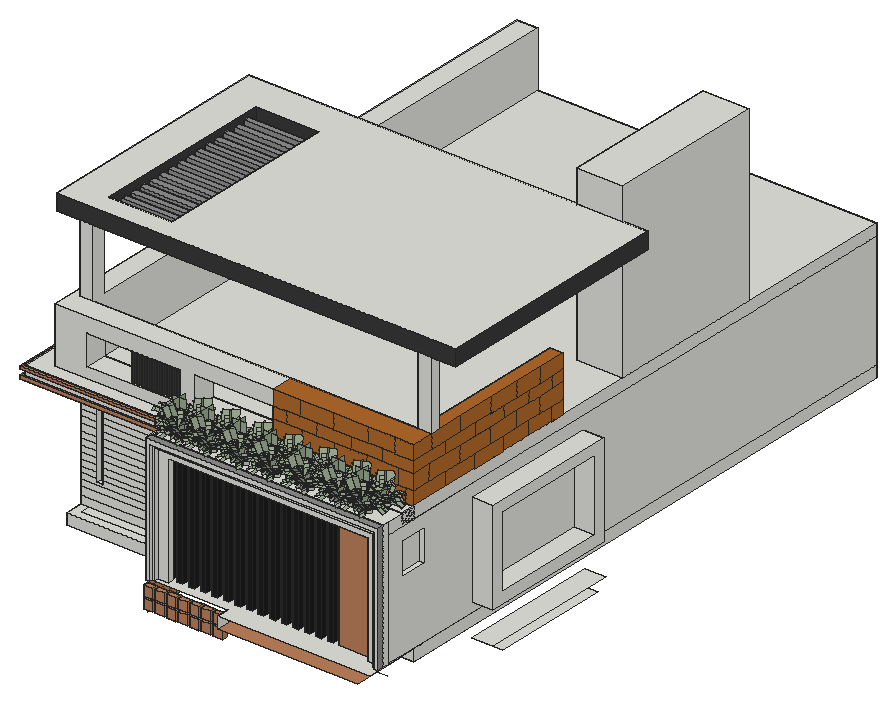
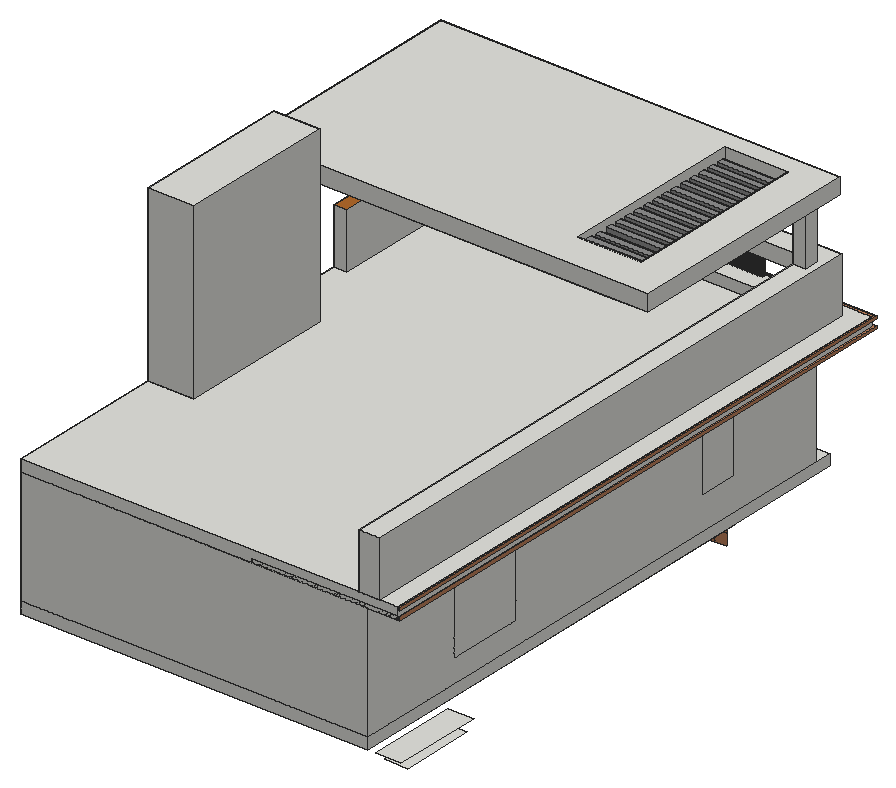
# SketchUp Ruby script. Lengths in inches.
U = 1.inch
M = Sketchup.active_model
def pt(a) = Geom::Point3d.new(a.map { |v| v * U })
def face(e, loops, mat)
  f = e.add_face(loops[0].map { |a| pt(a) })
  loops[1..].each { |l| e.add_face(l.map { |a| pt(a) }).erase! }
  f.material = f.back_material = mat if mat
  f
end
# faces: each face lists its corners as indices into pts; further lists are holes
def faces(e, pts, list, mat = nil) = list.each { |f| face(e, (f[0].is_a?(Array) ? f : [f]).map { |l| l.map { |i| pts[i] } }, mat) }
# xy, xz, yz: faces in a plane at the given z, y or x. An outline is a flat list of corners, or four numbers for a rectangle; further outlines are holes
def ring(l) = l.size == 4 ? [[l[0], l[1]], [l[2], l[1]], [l[2], l[3]], [l[0], l[3]]] : l.each_slice(2).to_a
def flat(e, list, mat, &to3) = list.each { |f| face(e, (f[0].is_a?(Array) ? f : [f]).map { |l| ring(l).map { |u, v| to3.(u, v) } }, mat) }
def xy(e, z, list, mat = nil) = flat(e, list, mat) { |x, y| [x, y, z] }
def xz(e, y, list, mat = nil) = flat(e, list, mat) { |x, z| [x, y, z] }
def yz(e, x, list, mat = nil) = flat(e, list, mat) { |y, z| [x, y, z] }
def lines(e, pts, list) = list.each { |a, b| e.add_line(pt(pts[a]), pt(pts[b])) }
# prism: a flat outline (further loops are holes) pulled along v
def prism(e, loops, v, mat = nil)
  f = face(e, loops, mat); d = Geom::Vector3d.new(v.map { |x| x * U })
  f.pushpull(f.normal.samedirection?(d) ? d.length : -d.length)
end
def box(e, o, s, mat = nil) = prism(e, [[o, [o[0] + s[0], o[1], o[2]], [o[0] + s[0], o[1] + s[1], o[2]], [o[0], o[1] + s[1], o[2]]]], [0, 0, s[2]], mat)
def at(x, y, z, deg = 0) = Geom::Transformation.translation(pt([x, y, z])) * Geom::Transformation.rotation(ORIGIN, Z_AXIS, deg.degrees)
def axes(o, x, y, z) = Geom::Transformation.new([*x, 0, *y, 0, *z, 0, *pt(o).to_a, 1])
def part(name) = M.definitions.add(name)
# library, detail: a bought-in or finely detailed component or shape, given as its bounding box
def library(name, o, s) = part(name).tap { |d| box(d.entities, o, s) }
def detail(e, o, s) = box(e.add_group.entities, o, s)
def put(e, d, t, mat = nil) = e.add_instance(d, t).tap { |i| i.material = mat if mat }
def group(e, t, mat = nil) = e.add_group.tap { |g| g.transformation = t; g.material = mat if mat }.entities
root = M.entities
M.materials.add("[Color M04]").color = [142, 142, 142]
M.materials.add("[Color M07]").color = [58, 58, 58]
M.materials.add("[Color M08]").color = [30, 30, 30]
M.materials.add("[Wood Bamboo]").color = [177, 105, 43]
M.materials.add("[Wood Veneer 02]").color = [190, 128, 91]
M.materials.add("hymenocallis littoralis").color = [156, 172, 146]
c1 = part("グループ\#88")
detail(c1.entities,[0,0,0],[11.8125,11.8125,1.69])
c2 = part("CL OL251733")
put(c2.entities,c1,axes([4.91,11.8125,72.56],[1,0,0],[0,-1,0],[0,0,-1]))
c3 = part("Group\#48")
box(c3.entities,[0,0,0],[5.9375,5.0625,120])
c4 = part("Group\#856")
xy(c4.entities,7.38,[[0,0,5.5,15.91]],"hymenocallis littoralis")
p = [[5.5,28.78,0],[5.5,26.79,3.44],[0,26.79,3.44],[0,28.78,0],[0,23.75,6],[5.5,23.75,6],
  [0,15.91,7.38],[5.5,15.91,7.38]]
faces(c4.entities,p,[[0,1,2,3],[4,2,1,5],[6,4,5,7]],"hymenocallis littoralis")
c5 = part("Group\#854")
xy(c5.entities,7.38,[[0,0,5.5,15.91],[0,15.91,5.5,23.87]],"hymenocallis littoralis")
p = [[5.5,31.07,4.3],[5.5,27.74,6.47],[0,27.74,6.47],[0,31.07,4.3],[0,23.87,7.38],[5.5,23.87,7.38]]
faces(c5.entities,p,[[0,1,2,3],[4,2,1,5]],"hymenocallis littoralis")
c6 = part("Group\#857")
xy(c6.entities,7.38,[[0,0,5.6,15.91]],"hymenocallis littoralis")
p = [[5.6,28.78,0],[5.6,26.79,3.44],[0,26.79,3.44],[0,28.78,0],[0,23.75,6],[5.6,23.75,6],
  [0,15.91,7.38],[5.6,15.91,7.38]]
faces(c6.entities,p,[[0,1,2,3],[4,2,1,5],[6,4,5,7]],"hymenocallis littoralis")
c7 = part("Group\#855")
put(c7.entities,c5,axes([6.09,8.57,-0.52],[0.446,0.85617,0.26089],[-0.18444,-0.19731,0.96283],[0.87582,-0.47754,0.0699]))
put(c7.entities,c5,axes([6.29,7.28,-1.71],[0.37058,0.92707,-0.05667],[-0.32382,0.19004,0.99128],[0.87712,-0.32925,0.34964]))
put(c7.entities,c5,axes([11.04,16.14,-0.7],[1,0,0],[0,0.16628,1.02662],[0,-1.18456,0.19186]))
c8 = part("Group\#860")
put(c8.entities,c4,axes([24.57,32.05,-1.76],[0.9552,-0.22102,-0.19681],[0.4036,0.95545,0.88585],[-0.00568,-0.67859,0.7345]))
put(c8.entities,c4,axes([23.95,29.24,-2.4],[0,1,0],[-0.76041,0,0.64945],[0.64945,0,0.76041]))
put(c8.entities,c4,axes([24.22,24.72,-0.48],[-0.70711,0.70711,0],[-0.32757,-0.32757,0.80237],[0.61237,0.61237,0.5]))
put(c8.entities,c5,axes([20.66,37.22,-0.63],[1.12361,0.03262,0.39091],[-0.43499,0.29739,0.78777],[0.09852,-1.27434,0.37535]))
put(c8.entities,c4,axes([28.75,24.45,-2.4],[-1,0,0],[0,-0.76041,0.64945],[0,0.64945,0.76041]))
put(c8.entities,c6,axes([30.4,30.98,-3.7],[0.65676,-0.72002,0.22414],[0.55667,0.66341,0.5],[-0.50871,-0.20361,0.83652]))
put(c8.entities,c6,axes([32.41,29.61,-3.7],[0.04029,-0.97372,0.22414],[0.85287,0.15038,0.5],[-0.52057,0.17102,0.83652]))
put(c8.entities,c4,axes([31.89,25.85,-1.76],[-0.92056,0.33739,-0.19681],[-0.5186,-0.89824,0.88585],[0.08952,0.67268,0.7345]))
put(c8.entities,c4,axes([25.55,34.78,-0.48],[0.86603,0.5,0],[-0.25,0.43301,0.86603],[0.43301,-0.75,0.5]))
put(c8.entities,c6,axes([20.4,16.9375,-8.07],[-0.70711,0.70711,0],[-0.35754,-0.35754,0.65422],[1.3987,1.3987,1.52882]))
put(c8.entities,c4,axes([32.86,34.14,-0.48],[0.76604,-0.64279,0],[0.32139,0.38302,0.86603],[-0.55667,-0.66341,0.5]))
put(c8.entities,c4,axes([27.15,34.7,-0.1],[0.82472,-0.17528,-0.53769],[0.53769,0.53769,0.64945],[0.17528,-0.82472,0.53769]))
put(c8.entities,c4,axes([33.58,28.77,-2.4],[0,-1,0],[0.76041,0,0.64945],[-0.64945,0,0.76041]))
put(c8.entities,c4,axes([26.43,23.87,-2.81],[-0.75126,0.04415,0.65853],[0.53769,-0.53769,0.64945],[0.38276,0.84199,0.3802]))
put(c8.entities,c4,axes([28.78,23.98,-2.4],[-1,0,0],[0,-0.76041,0.64945],[0,0.64945,0.76041]))
put(c8.entities,c4,axes([25.39,25.38,-2.4],[-0.70711,0.70711,0],[-0.53769,-0.53769,0.64945],[0.45923,0.45923,0.76041]))
put(c8.entities,c4,axes([27.32,21.63,-0.1],[-0.45923,0.70711,-0.53769],[-0.76041,0,0.64945],[0.45923,0.70711,0.53769]))
put(c8.entities,c4,axes([25.17,27.625,-1.76],[0.56416,0.80187,-0.19681],[-0.66673,0.66673,0.80532],[0.62659,-0.26057,0.7345]))
put(c8.entities,c6,axes([27.59,27.04,-3.96],[-0.8993,-0.06127,0.43301],[0.2962,-0.8138,0.5],[0.32175,0.57791,0.75]))
put(c8.entities,c6,axes([26.98,24.5,-3.18],[-0.5,0.86603,0],[-0.75,-0.43301,0.5],[0.43301,0.25,0.86603]))
put(c8.entities,c6,axes([24.55,27.74,-3.7],[0.29517,0.92878,0.22414],[-0.85287,0.15038,0.5],[0.43068,-0.33875,0.83652]))
put(c8.entities,c6,axes([24.26,29.8,-3.18],[0.76604,0.64279,0],[-0.47317,0.5639,0.425],[0.32139,-0.38302,0.86603]))
put(c8.entities,c6,axes([25.98,32.46,-3.18],[1,0,0],[0,0.86603,0.5],[0,-0.5,0.86603]))
put(c8.entities,c4,axes([28.78,33.57,-2.4],[1,0,0],[0,0.76041,0.64945],[0,-0.64945,0.76041]))
put(c8.entities,c7,at(14.99,21.38,2.5))
put(c8.entities,c5,axes([34.63,26.34,-1.46],[-0.70089,-0.70877,0.07994],[0.4756,-0.38088,0.79293],[-0.53156,0.59378,0.60405]))
put(c8.entities,c5,axes([28.14,16.92,1.8125],[-1.19719,0.6912,0],[-0.09607,-0.16641,0.94244],[0.68444,1.18549,0.17613]))
put(c8.entities,c5,axes([31.5625,35.84,0.97],[0.66765,-1.1564,0.35779],[0.04445,0.30732,0.91033],[-1.20828,-0.64496,0.17012]))
put(c8.entities,c5,axes([38.94,22.51,0.89],[-0.97932,-0.67164,-0.05202],[0.27787,-0.41401,0.90999],[-0.85985,0.93577,0.32097]))
put(c8.entities,c5,axes([38.44,21.09,1.98],[-1.02864,-0.54856,0.2395],[0.33481,0.06999,0.88388],[-0.77261,1.08328,0.06417]))
put(c8.entities,c6,axes([35.02,30.51,-1.3],[-0.17365,-0.98481,0],[0.60224,-0.10619,0.79122],[-0.7792,0.13739,0.61153]))
put(c8.entities,c6,axes([29.41,22.33,-1.3],[-0.93969,0.34202,0],[-0.20915,-0.57465,0.79122],[0.27061,0.74351,0.61153]))
put(c8.entities,c5,axes([19.64,36,-1.62],[1.18194,0.09546,0.08234],[-0.14377,0.68823,0.76313],[0.21457,-1.1326,0.62386]))
put(c8.entities,c6,axes([24.25,24.14,-1.3],[-0.34202,0.93969,0],[-0.57465,-0.20915,0.79122],[0.74351,0.27061,0.61153]))
put(c8.entities,c6,axes([25.98,34.61,-1.3],[1,0,0],[0,0.61153,0.79122],[0,-0.79122,0.61153]))
put(c8.entities,c6,axes([31.16,34.41,-1.64],[0.56518,-0.80224,-0.19234],[0.73413,0.34233,0.72935],[-0.47639,-0.50772,0.71782]))
put(c8.entities,c6,axes([40.52,26.84,-5.82],[-0.42262,-0.90631,0],[0.48019,-0.22391,0.68552],[-1.43418,0.66877,1.22305]))
put(c8.entities,c4,axes([29.86,38.42,-1.01],[0.89064,-0.37013,0.26413],[-0.03924,0.63286,1.01918],[-0.45353,-0.76487,0.45748]))
put(c8.entities,c4,axes([29.34,22.4,-0.48],[-0.99619,-0.08716,0],[0.04358,-0.4981,0.86603],[-0.07548,0.86273,0.5]))
c9 = part("Group\#858")
xz(c9.entities,10.07,[[9.07,0,10.07,31.01],[0,31.01,0,45.12,20.13,45.12,20.13,31.01,10.07,31.01,10.07,32.58,9.07,32.58,9.07,31.01]],"hymenocallis littoralis")
yz(c9.entities,10.07,[[0,31.01,20.13,45.12]],"hymenocallis littoralis")
p = [[9.57,9.2,0],[10.07,10.07,0],[10.07,10.07,31.01],[10.07,10.07,32.58],[9.57,9.2,32.58]]
faces(c9.entities,p,[[0,1,2,3,4]],"hymenocallis littoralis")
c10 = part("cây lá nắng")
put(c10.entities,c8,axes([49.26,-2.75,0],[0.63109,0.63109,0],[-0.63109,0.63109,0],[0,0,0.935]))
g1 = group(c10.entities,at(26.6,-8.68,0))
put(g1,c4,axes([-4.72,35.73,-1.65],[0.74231,0.46334,-0.18402],[-0.34827,0.85768,0.82827],[0.42467,-0.43184,0.68675]))
put(g1,c4,axes([-3.34,33.57,-2.24],[-0.63109,0.63109,0],[-0.47989,-0.47989,0.60723],[0.40986,0.40986,0.71098]))
put(g1,c4,axes([-0.3125,30.89,-0.45],[-0.8925,0,0],[0,-0.41345,0.75022],[0,0.77293,0.4675]))
put(g1,c5,axes([-10.79,39.66,-0.59],[0.68852,0.72969,0.3655],[-0.4622,-0.08684,0.73657],[0.86641,-0.74205,0.35095]))
put(g1,c4,axes([2.71,33.57,-2.24],[-0.63109,-0.63109,0],[0.47989,-0.47989,0.60723],[-0.40986,0.40986,0.71098]))
put(g1,c6,axes([-0.37,38.74,-3.46],[0.86887,-0.03992,0.20957],[-0.06737,0.76999,0.4675],[-0.19255,-0.44954,0.78214]))
put(g1,c6,axes([1.76,39.14,-3.46],[0.63993,-0.58908,0.20957],[0.44333,0.63315,0.4675],[-0.43646,-0.2206,0.78214]))
put(g1,c4,axes([3.81,36.4375,-1.65],[-0.79389,-0.36803,-0.18402],[0.23959,-0.89415,0.82827],[-0.36803,0.48102,0.68675]))
put(g1,c4,axes([-5.83,38.07,-0.45],[0.231,0.86209,0],[-0.43104,0.1155,0.80973],[0.74659,-0.20005,0.4675]))
put(g1,c6,axes([2.18,23.5625,-7.55],[-0.8925,0,0],[0,-0.45128,0.6117],[0,1.76542,1.42944]))
put(g1,c4,axes([-0.8125,42.28,-0.45],[0.8891,0.07779,0],[-0.03889,0.44455,0.80973],[0.06737,-0.76999,0.4675]))
put(g1,c4,axes([-4.76,39.03,-0.09],[0.63109,0.40986,-0.50274],[0,0.67866,0.60723],[0.63109,-0.40986,0.50274]))
put(g1,c4,axes([3.03,39.35,-2.24],[0.63109,-0.63109,0],[0.47989,0.47989,0.60723],[-0.40986,-0.40986,0.71098]))
put(g1,c4,axes([1.61,31.74,-2.625],[-0.50198,-0.44625,0.61573],[0.67866,0,0.60723],[-0.28982,0.77293,0.35549]))
put(g1,c4,axes([3.03,33.3,-2.24],[-0.63109,-0.63109,0],[0.47989,-0.47989,0.60723],[-0.40986,0.40986,0.71098]))
put(g1,c4,axes([0.01,32.04,-2.24],[-0.8925,0,0],[0,-0.67866,0.60723],[0,0.57963,0.71098]))
put(g1,c4,axes([3.59,30.89,-0.09],[-0.73607,0.15643,-0.50274],[-0.47989,-0.47989,0.60723],[-0.15643,0.73607,0.50274]))
put(g1,c4,axes([-1.55,33.32,-1.65],[-0.15002,0.86209,-0.18402],[-0.84154,0,0.75297],[0.55988,0.231,0.68675]))
put(g1,c6,axes([0.35,34.48,-3.71],[-0.52887,-0.60621,0.40487],[0.70051,-0.32665,0.4675],[-0.16166,0.56777,0.70125]))
put(g1,c6,axes([2.61,39.13,-1.74],[-0.86209,0.231,0],[-0.23031,-0.85954,0.15531],[0.03162,0.11799,0.91645]))
put(g1,c6,axes([-2.02,33,-3.46],[-0.39986,0.77243,0.20957],[-0.63315,-0.44333,0.4675],[0.48558,0.05802,0.78214]))
put(g1,c6,axes([-3.49,34.12,-2.97],[0.07779,0.8891,0],[-0.65449,0.05726,0.39737],[0.44455,-0.03889,0.80973]))
put(g1,c6,axes([-4.09,36.88,-2.97],[0.63109,0.63109,0],[-0.54654,0.54654,0.4675],[0.31555,-0.31555,0.80973]))
put(g1,c4,axes([-3.02,39.35,-2.24],[0.63109,0.63109,0],[-0.47989,0.47989,0.60723],[0.40986,-0.40986,0.71098]))
put(g1,c7,axes([-4.03,22.95,2.33],[0.63109,0.63109,0],[-0.63109,0.63109,0],[0,0,0.935]))
put(g1,c5,axes([5.24,38.48,-1.37],[0.00497,-0.88963,0.07474],[0.54052,0.05978,0.74139],[-0.71019,0.03927,0.56479]))
put(g1,c5,axes([7.08,28.4375,1.7],[-1.19175,-0.31933,0],[0.04439,-0.16565,0.88118],[-0.31621,1.1801,0.16468]))
put(g1,c5,axes([-2.7,42.54,0.91],[1.15114,-0.30845,0.33454],[-0.1659,0.22199,0.85115],[-0.3555,-1.16957,0.15907]))
put(g1,c5,axes([10.37,38.78,0.83],[-0.19417,-1.04191,-0.04864],[0.43664,-0.08592,0.85084],[-1.1332,0.04791,0.30011]))
put(g1,c5,axes([10.95,37.5625,1.85],[-0.30298,-0.99536,0.22393],[0.16713,0.25547,0.82643],[-1.17124,0.19607,0.06]))
put(g1,c6,axes([2.84,41.36,-1.22],[0.51192,-0.73109,0],[0.44708,0.31305,0.73979],[-0.57846,-0.40504,0.57178]))
put(g1,c6,axes([4.47,32.65,-1.22],[-0.80888,-0.37719,0],[0.23066,-0.49465,0.73979],[-0.29844,0.64,0.57178]))
put(g1,c5,axes([-10.32,35.12,-1.51],[0.68567,0.80616,0.07699],[-0.52507,0.3436,0.71352],[0.85019,-0.57936,0.58331]))
put(g1,c6,axes([0.07,30.54,-1.22],[-0.80888,0.37719,0],[-0.23066,-0.49465,0.73979],[0.29844,0.64,0.57178]))
put(g1,c6,axes([-5.45,38.24,-1.22],[0.63109,0.63109,0],[-0.38593,0.38593,0.73979],[0.49934,-0.49934,0.57178]))
put(g1,c6,axes([-2.05,41.38,-1.53],[0.86296,-0.14961,-0.17984],[0.24726,0.67935,0.68194],[0.01977,-0.62107,0.67116]))
put(g1,c6,axes([8.63,42.51,-5.4375],[0.30525,-0.83868,0],[0.44435,0.16173,0.64096],[-1.32716,-0.48305,1.14356]))
put(g1,c4,axes([-5.4,43.09,-0.94],[0.79566,0.32849,0.24696],[-0.42416,0.37462,0.95293],[0.19648,-0.76892,0.42774]))
put(g1,c4,axes([4.38,32.65,-0.45],[-0.57369,-0.68369,0],[0.34185,-0.28684,0.80973],[-0.5921,0.49683,0.4675]))
put(g1,c6,axes([-2,33.84,-0.15],[-0.24601,0.85793,0],[-0.85539,-0.24528,0.15531],[0.11742,0.03367,0.91645]))
put(g1,c6,axes([0.17,30.83,-4.47],[-0.24601,0.85793,0],[-0.85539,-0.24528,0.15531],[0.11742,0.03367,0.91645]))
put(g1,c6,axes([-1.97,32.18,-4.47],[0.58524,0.67383,0],[-0.67184,0.58351,0.15531],[0.09222,-0.0801,0.91645]))
put(g1,c6,axes([-2,34.71,-4.47],[0.88392,-0.12346,0],[0.12309,0.88131,0.15531],[-0.0169,-0.12098,0.91645]))
put(g1,c6,axes([0.11,36.12,-4.47],[0.37822,-0.8084,0],[0.80601,0.37711,0.15531],[-0.11064,-0.05177,0.91645]))
put(c10.entities,c9,axes([29.71,14.29,6.94],[0.425,0.73612,0],[-0.6771,0.39092,-0.33349],[-0.26859,0.15507,0.72712]))
put(c10.entities,c9,axes([42.0625,26.12,6.94],[0.85,0,0],[0,0.78185,-0.33349],[0,0.33349,0.78185]))
put(c10.entities,c8,axes([7.3125,23.0625,0],[0.8925,0,0],[0,0.8925,0],[0,0,0.935]))
put(c10.entities,c9,axes([24.4375,40.23,2.05],[0.85,0,0],[0,0.85,0],[0,0,0.85]))
c11 = part("Planting 101")
put(c11.entities,c10,axes([21.34,32.96,-4.59],[0,-0.71,0],[-0.71,0,0],[0,0,0.71]))
c12 = part("Group\#49")
box(c12.entities,[0,0,0],[3.3125,2.6875,31.375])
c13 = part("Group\#50")
box(c13.entities,[0,0,0],[6.8125,4.9375,68.4375])
xy(root,231.53,[[394.0625,149.62,416.125,272.62]])
xy(root,235.36,[[7.8125,565.56,31.8125,641.91]])
xy(root,240.5,[[394.0625,137.15,416.125,283.4]])
xy(root,244.31,[[7.8125,556.61,34.0625,650.86]])
xy(root,251.875,[[171.15,61.36,187.02,184.55]])
xy(root,252,[[[387.09,61.62,394.0625,61.62,394.0625,661.36,34.0625,661.36,34.0625,184.55,387.09,184.55],[43.0625,193.55,385.0625,652.36]]])
xy(root,252,[[236.46,4.36,381.58,61.36]],"[Wood Veneer 02]")
xy(root,264,[[[236.46,4.36,394.0625,4.36,394.0625,14.86,389.97,14.86,389.97,17.49,386.8,17.49,386.8,21.55,378.29,21.55,378.29,27.62,394.0625,27.62,394.0625,184.55,385.0625,184.55,385.0625,70.36,160.65,70.36,160.65,27.62,171.65,27.62,171.65,21.55,160.36,21.55,160.36,17.49,157.48,17.49,157.48,17.17,236.46,17.17],[343.16,27.62,378.29,36.68]],[153.47,14.86,157.48,17.17],[34.0625,61.36,153.47,61.36,153.47,70.36,43.0625,70.36,43.0625,79.99,34.0625,79.99],[43.0625,70.36,153.47,79.99],[160.65,70.36,385.0625,184.55],
  [[34.0625,79.99,153.47,79.99,153.47,87.06,43.0625,87.06,43.0625,184.55,394.0625,184.55,394.0625,661.36,34.0625,661.36],[43.0625,193.55,385.0625,652.36]],[43.0625,87.06,153.47,184.55],[43.0625,193.55,385.0625,652.36]])
xy(root,274.55,[[394.0625,136.625,416.125,280.1875]])
xy(root,286.26,[[394.0625,148.1,416.125,268.91]])
xy(root,289.77,[[50.92,79.99,56.92,84.62]])
xy(root,337.08,[[388.6875,46.5625,394.0625,75.3125]])
xy(root,360.2,[[394.0625,148.1,416.125,268.91]])
xy(root,370.58,[[388.6875,46.5625,394.0625,75.3125]])
xy(root,371.42,[[394.0625,136.625,416.125,280.1875]])
xy(root,373.77,[[50.92,79.99,56.92,84.62]])
xy(root,379.125,[[171.65,21.55,378.29,27.62],[343.16,27.62,378.29,36.68]])
xy(root,383.75,[[160.65,27.62,394.0625,61.36],[153.47,61.36,160.65,184.55]])
xy(root,384,[[34.0625,79.99,153.47,79.99,153.47,87.06,43.0625,87.06,43.0625,184.55,153.47,184.55,153.47,193.55,43.0625,193.55,43.0625,652.36,153.47,652.36,153.47,661.36,34.0625,661.36],[43.0625,87.06,153.47,184.55],[153.47,184.55,394.0625,184.55,394.0625,661.36,153.47,661.36,153.47,652.36,385.0625,652.36,385.0625,193.55,153.47,193.55],[43.0625,193.55,153.47,652.36]])
xy(root,384,[[0,43.99,0,661.36,34.0625,661.36,34.0625,79.99,153.47,79.99,153.47,43.99]],"[Wood Veneer 02]")
xy(root,387.21,[[0,43.99,153.47,661.36]],"[Wood Veneer 02]")
xy(root,387.45,[[160.36,17.49,386.8,21.55]])
xy(root,390.95,[[157.48,14.86,389.97,17.49],[157.48,17.49,389.97,21.55]])
xy(root,393.1875,[[0,43.99,0,661.36,2.3125,661.36,2.3125,46.74,153.47,46.74,153.47,43.99]],"[Wood Veneer 02]")
xy(root,396,[[153.47,21.55,394.0625,61.36],[21.4375,61.36,21.4375,661.36,42.41,661.36,42.41,84.53,380.375,84.53,380.375,255.3,394.0625,255.3,394.0625,61.36],[346.5,333.07,394.0625,495.82]])
xy(root,396,[[153.47,14.86,394.0625,21.55]],"[Color M04]")
xy(root,396,[[0,43.99,153.47,43.99,153.47,46.74,2.3125,46.74,2.3125,661.36,0,661.36]],"[Wood Veneer 02]")
xy(root,406.81,[[55.15,61.36,151.97,84.53]])
xy(root,408.1,[[167.29,61.36,247.91,84.53]])
xy(root,438.24,[[55.15,61.36,151.97,84.53]])
xy(root,438.29,[[167.29,61.36,247.91,84.53]])
xy(root,453.625,[[21.4375,61.36,247.91,61.36,247.91,84.53,29.09,84.53,29.09,98.85,42.41,98.85,42.41,661.36,21.4375,661.36]])
xy(root,453.625,[[247.91,61.36,394.0625,84.53],[380.375,94.4,394.0625,255.3]],"[Wood Bamboo]")
xy(root,524.3125,[[29.09,84.53,42.41,98.85],[380.375,84.53,394.0625,94.4],[394.0625,104.68,398.6,108.15]])
xy(root,524.3125,[[5.78,84.53,29.09,108.78],[42.41,84.53,42.41,108.78,43.2,108.78,43.2,104.55,108.45,104.55,108.45,294.99,47.66,294.99,47.66,333.07,419.375,333.07,419.375,108.15,398.6,108.15,398.6,321.37,128.79,321.37,128.79,104.68,394.0625,104.68,394.0625,94.4,380.375,94.4,380.375,84.53],[394.0625,84.53,394.0625,104.68,398.6,104.68,398.6,108.15,419.375,108.15,419.375,84.53],[29.09,98.85,29.09,108.78,5.78,108.78,5.78,333.07,47.66,333.07,47.66,294.99,43.2,294.99,43.2,108.78,42.41,108.78,42.41,98.85]],"[Color M07]")
xy(root,524.3125,[[128.79,104.68,128.79,321.37,398.6,321.37,398.6,108.15,394.0625,108.15,394.0625,104.68]],"[Wood Bamboo]")
xy(root,541.25,[[[5.78,84.53,419.375,333.07],[43.2,104.55,108.45,294.99]]])
xy(root,575.0625,[[346.5,333.07,394.0625,495.82]])
xz(root,14.86,[[153.47,264,157.48,264,157.48,390.95,389.97,390.95,389.97,264,394.0625,264,394.0625,396,153.47,396]])
xz(root,17.49,[[157.48,264,160.36,264,160.36,387.45,386.8,387.45,386.8,264,389.97,264,389.97,390.95,157.48,390.95]])
xz(root,21.55,[[153.47,264,153.47,396,394.0625,396,394.0625,264,389.97,264,389.97,390.95,157.48,390.95,157.48,264],[160.36,264,171.65,264,171.65,379.125,378.29,379.125,378.29,264,386.8,264,386.8,387.45,160.36,387.45]])
xz(root,27.62,[[160.65,264,171.65,383.75],[378.29,264,394.0625,383.75],[171.65,379.125,378.29,383.75]])
xz(root,27.62,[[343.16,264,378.29,379.125]],"[Wood Veneer 02]")
xz(root,36.68,[[343.16,264,378.29,379.125]])
xz(root,43.99,[[0,384,153.47,387.21],[0,393.1875,153.47,396]],"[Wood Veneer 02]")
xz(root,46.5625,[[388.6875,337.08,394.0625,370.58]])
xz(root,46.74,[[2.3125,393.1875,153.47,396]])
xz(root,61.36,[[153.47,383.75,394.0625,396],[[21.4375,396,247.91,396,247.91,408.1,167.29,408.1,167.29,438.29,247.91,438.29,247.91,453.625,21.4375,453.625],[55.15,406.81,151.97,438.24]]])
xz(root,61.36,[[247.91,396,262.97,410.29],[262.97,396,294.85,410.29],[294.85,396,328.35,410.29],[328.35,396,361.21,410.29],[361.21,396,385.72,410.29],
  [385.72,396,394.0625,410.29],[247.91,410.29,278.02,426.29],[278.02,410.29,311.68,426.29],[311.68,410.29,345.03,426.29],[345.03,410.29,377.38,426.29],
  [377.38,410.29,394.0625,426.29],[247.91,426.29,262.05,438.29],[262.05,426.29,293.99,438.29],[293.99,426.29,329.36,438.29],[329.36,426.29,360.7,438.29],
  [360.7,426.29,394.0625,438.29],[247.91,438.29,276.1875,453.625],[276.1875,438.29,311.79,453.625],[311.79,438.29,346.93,453.625],[346.93,438.29,374.48,453.625],
  [374.48,438.29,394.0625,453.625]],"[Wood Bamboo]")
xz(root,75.3125,[[388.6875,337.08,394.0625,370.58]])
xz(root,79.99,[[34.0625,264,153.47,272.5],[34.0625,272.5,153.47,280.25],[34.0625,280.25,153.47,287.0625],[34.0625,287.0625,153.47,287.0625,153.47,293.1875,56.92,293.1875,56.92,289.77,50.92,289.77,50.92,293.1875,34.0625,293.1875],[34.0625,293.1875,50.92,299.125],
  [56.92,293.1875,153.47,299.125],[34.0625,299.125,50.92,305.5],[56.92,299.125,153.47,305.5],[34.0625,305.5,50.92,312.1875],[56.92,305.5,153.47,312.1875],
  [34.0625,312.1875,50.92,318.5625],[56.92,312.1875,153.47,318.5625],[34.0625,318.5625,50.92,325.0625],[56.92,318.5625,153.47,325.0625],[34.0625,325.0625,50.92,331.8125],
  [56.92,325.0625,153.47,331.8125],[34.0625,331.8125,50.92,339],[56.92,331.8125,153.47,339],[34.0625,339,50.92,346.125],[56.92,339,153.47,346.125],
  [34.0625,346.125,50.92,352.125],[56.92,346.125,153.47,352.125],[34.0625,352.125,50.92,358.5625],[56.92,352.125,153.47,358.5625],[34.0625,358.5625,50.92,364.5625],
  [56.92,358.5625,153.47,364.5625],[34.0625,364.5625,50.92,371.1875],[56.92,364.5625,153.47,371.1875],[34.0625,371.1875,50.92,371.1875,50.92,373.77,56.92,373.77,56.92,371.1875,153.47,371.1875,153.47,377.1875,34.0625,377.1875],[34.0625,377.1875,153.47,384]])
xz(root,84.53,[[[42.41,396,380.375,453.625],[55.15,406.81,151.97,438.24],[167.29,408.1,247.91,438.29]],[29.09,453.625,42.41,524.3125],[380.375,453.625,394.0625,524.3125]])
xz(root,84.53,[[5.78,524.3125,419.375,541.25]],"[Color M07]")
xz(root,84.62,[[50.92,289.77,56.92,373.77]])
xz(root,87.06,[[43.0625,264,153.47,384]])
xz(root,94.4,[[380.375,453.625,394.0625,524.3125]])
xz(root,98.85,[[29.09,453.625,42.41,524.3125]])
xz(root,104.55,[[43.2,524.3125,108.45,541.25]])
xz(root,136.625,[[394.0625,274.55,416.125,371.42]])
xz(root,148.1,[[394.0625,286.26,416.125,360.2]])
xz(root,184.55,[[43.0625,264,153.47,384],[153.47,264,160.65,383.75],[160.65,264,385.0625,384],[153.47,383.75,160.65,384]])
xz(root,184.55,[[43.0625,228.9,55.05,240.9],[55.05,228.9,78.83,240.9],[78.83,228.9,103.16,240.9],[103.16,228.9,130.75,240.9],[130.75,228.9,158.47,240.9],
  [158.47,228.9,171.15,240.9],[43.0625,240.9,67.04,252],[67.04,240.9,90.61,252],[90.61,240.9,115.71,252],[115.71,240.9,145.79,252]],"[Wood Veneer 02]")
xz(root,193.55,[[43.0625,264,385.0625,384]])
xz(root,255.3,[[380.375,396,394.0625,453.625]])
xz(root,268.91,[[394.0625,286.26,416.125,360.2]])
xz(root,280.1875,[[394.0625,274.55,416.125,371.42]])
xz(root,294.99,[[43.2,524.3125,108.45,541.25]],"[Color M07]")
xz(root,333.07,[[346.5,396,394.0625,524.3125],[5.78,524.3125,346.5,541.25],[346.5,524.3125,394.0625,541.25],[394.0625,524.3125,419.375,541.25],[346.5,541.25,394.0625,575.0625]])
xz(root,495.82,[[346.5,396,394.0625,575.0625]])
xz(root,652.36,[[43.0625,264,385.0625,384]])
xz(root,661.36,[[34.0625,264,394.0625,384],[0,384,153.47,387.21],[0,393.1875,2.3125,396],[21.4375,396,42.41,453.625]])
yz(root,0,[[43.99,384,661.36,387.21],[43.99,393.1875,661.36,396]],"[Wood Veneer 02]")
yz(root,2.3125,[[46.74,393.1875,661.36,396]])
yz(root,5.78,[[84.53,524.3125,333.07,541.25]])
yz(root,21.4375,[[61.36,396,661.36,453.625]])
yz(root,29.09,[[84.53,453.625,98.85,524.3125]])
yz(root,34.0625,[[[79.99,264,661.36,384],[468.8125,287.01,548.875,356.01],[186.29,297.7,227.54,354.52]],[468.8125,287.01,548.875,356.01],[186.29,297.7,227.54,354.52]])
yz(root,42.41,[[84.53,396,661.36,396,661.36,453.625,98.85,453.625,98.85,524.3125,84.53,524.3125]])
yz(root,43.0625,[[87.06,264,184.55,384],[193.55,264,652.36,384]])
yz(root,43.2,[[104.55,524.3125,294.99,541.25]],"[Color M07]")
yz(root,50.92,[[79.99,289.77,84.62,373.77]])
yz(root,55.15,[[61.36,406.81,84.53,438.24]])
yz(root,56.92,[[79.99,289.77,84.62,373.77]])
yz(root,108.45,[[104.55,524.3125,294.99,541.25]])
yz(root,151.97,[[61.36,406.81,84.53,438.24]])
yz(root,153.47,[[21.55,264,21.55,396,43.99,396,43.99,393.1875,46.74,393.1875,46.74,396,61.36,396,61.36,387.21,43.99,387.21,43.99,384,61.36,384,61.36,383.75,79.99,383.75,79.99,264],[79.99,264,87.06,383.75],[87.06,264,184.55,383.75],[79.99,383.75,87.06,384],[43.99,384,61.36,387.21],
  [61.36,384,661.36,387.21]])
yz(root,153.47,[[14.86,264,21.55,396]],"[Color M04]")
yz(root,153.47,[[17.17,233.2,23.52,240.43],[23.52,233.2,39.92,240.43],[39.92,233.2,54.27,240.43],[54.27,233.2,61.36,240.43],[17.17,240.43,32.67,247.3],
  [32.67,240.43,47.17,247.3],[47.17,240.43,61.36,247.3],[17.17,247.3,25.69,255.65],[25.69,247.3,39.64,255.65],[39.64,247.3,54.71,255.65],
  [54.71,247.3,61.36,255.65],[17.17,255.65,34.22,264],[34.22,255.65,48.06,264],[48.06,255.65,61.36,264]],"[Wood Veneer 02]")
yz(root,157.48,[[14.86,264,17.49,390.95],[17.49,264,21.55,390.95]])
yz(root,160.36,[[17.49,264,21.55,387.45]])
yz(root,160.65,[[27.62,264,184.55,383.75]])
yz(root,167.29,[[61.36,408.1,84.53,438.29]])
yz(root,171.65,[[21.55,264,27.62,379.125]])
yz(root,236.46,[[4.36,252,17.17,264]])
yz(root,247.91,[[61.36,408.1,84.53,438.29]])
yz(root,343.16,[[27.62,264,36.68,379.125]],"[Wood Veneer 02]")
yz(root,346.5,[[333.07,396,495.82,575.0625]])
yz(root,378.29,[[21.55,264,27.62,379.125],[27.62,264,36.68,379.125]])
yz(root,378.88,[[27.88,253.06,27.62,383.68,61.36,383.75,184.55,384,184.82,253.375]])
yz(root,380.375,[[84.53,396,84.53,524.3125,94.4,524.3125,94.4,453.625,255.3,453.625,255.3,396]])
yz(root,385.0625,[[193.55,264,652.36,384]])
yz(root,386.8,[[17.49,264,21.55,387.45]])
yz(root,388.6875,[[46.5625,337.08,75.3125,370.58]])
yz(root,389.97,[[14.86,264,17.49,390.95]])
yz(root,394.0625,[[27.86,263.93,61.36,264,27.86,264],[21.55,264,27.62,396],[[27.86,264,661.36,264,661.36,384,184.55,384,61.36,383.75,27.62,383.68],[136.625,274.55,280.1875,371.42],[46.5625,337.08,75.3125,370.58]],[148.1,286.26,268.91,360.2],[27.62,383.75,61.36,396],
  [333.07,396,495.82,575.0625],[84.53,453.625,94.4,524.3125]])
yz(root,394.0625,[[14.86,264,21.55,396]],"[Color M04]")
yz(root,394.0625,[[61.36,396,101.46,410.29],[101.46,396,140.58,410.29],[140.58,396,176.96,410.29],[176.96,396,209.7,410.29],[209.7,396,240.25,410.29],
  [240.25,396,255.3,410.29],[61.36,410.29,81.49,426.29],[81.49,410.29,121.43,426.29],[121.43,410.29,159.72,426.29],[159.72,410.29,194.1875,426.29],
  [194.1875,410.29,225.2,426.29],[225.2,410.29,255.3,426.29],[61.36,426.29,101.625,438.29],[101.625,426.29,141.23,438.29],[141.23,426.29,178.22,438.29],
  [178.22,426.29,210.16,438.29],[210.16,426.29,240.25,438.29],[240.25,426.29,255.3,438.29],[61.36,438.29,84.53,453.625],[84.53,438.29,121.13,453.625],
  [121.13,438.29,161.33,453.625],[161.33,438.29,195.11,453.625],[195.11,438.29,225.2,453.625],[225.2,438.29,255.3,453.625]],"[Wood Bamboo]")
yz(root,416.125,[[[136.625,274.55,280.1875,371.42],[148.1,286.26,268.91,360.2]]])
yz(root,419.375,[[84.53,524.3125,333.07,541.25]],"[Color M07]")
p = [[378.88,184.55,384],[385.0625,184.55,384],[385.0625,184.82,253.375],[378.88,184.82,253.375],[394.0625,61.36,383.75],[378.88,61.36,383.75],
  [378.88,27.62,383.68],[394.0625,27.62,383.68],[394.0625,184.55,384],[394.0625,184.82,253.375],[378.88,27.88,253.06],[394.0625,27.88,253.06],
  [160.65,27.62,383.75],[153.47,27.62,383.75],[160.65,27.62,264],[153.47,27.62,264]]
faces(root,p,[[0,1,2,3],[4,5,6,7],[4,8,1,0,5]])
lines(root,p,[[9,2],[10,11],[12,13],[14,15]])
g2 = group(root,at(165.47,17.17,238.41))
box(g2,[0,-5.4375,0],[10,5.4375,10],"[Wood Veneer 02]")
g3 = group(root,at(153.47,17.17,238.41))
box(g3,[0,-5.4375,0],[10,5.4375,10],"[Wood Veneer 02]")
g4 = group(root,at(189.47,17.17,238.41))
box(g4,[0,-5.4375,0],[10,5.4375,10],"[Wood Veneer 02]")
g5 = group(root,at(213.47,17.17,238.41))
box(g5,[0,-5.4375,0],[10,5.4375,10],"[Wood Veneer 02]")
g6 = group(root,at(201.47,17.17,238.41))
box(g6,[0,-5.4375,0],[10,5.4375,10],"[Wood Veneer 02]")
g7 = group(root,at(177.47,17.17,238.41))
box(g7,[0,-5.4375,0],[10,5.4375,10],"[Wood Veneer 02]")
g8 = group(root,at(225.47,17.17,238.41))
box(g8,[0,-5.4375,0],[10,5.4375,10],"[Wood Veneer 02]")
put(root,c2,at(127.66,85.4,175.95))
put(root,c2,at(52.6,85.4,175.95))
put(root,c2,at(52.6,127.28,175.95))
put(root,c2,at(127.66,127.28,175.95))
put(root,c2,at(263.2,27.05,179.2))
put(root,c2,at(337.76,27.05,179.2))
g9 = group(root,at(153.47,17.17,250.41),"[Wood Veneer 02]")
box(g9,[0,-5.4375,0],[10,5.4375,10],"[Wood Veneer 02]")
g10 = group(root,at(165.47,17.17,250.41),"[Wood Veneer 02]")
box(g10,[0,-5.4375,0],[10,5.4375,10],"[Wood Veneer 02]")
g11 = group(root,at(177.47,17.17,250.41))
box(g11,[0,-5.4375,0],[10,5.4375,10],"[Wood Veneer 02]")
g12 = group(root,at(189.47,17.17,250.41))
box(g12,[0,-5.4375,0],[10,5.4375,10],"[Wood Veneer 02]")
g13 = group(root,at(201.47,17.17,250.41))
box(g13,[0,-5.4375,0],[10,5.4375,10],"[Wood Veneer 02]")
g14 = group(root,at(213.47,17.17,250.41))
box(g14,[0,-5.4375,0],[10,5.4375,10],"[Wood Veneer 02]")
g15 = group(root,at(225.47,17.17,250.41))
box(g15,[0,-5.4375,0],[10,5.4375,10],"[Wood Veneer 02]")
g16 = group(root,at(34.0625,661.36,252))
xy(g16,0,[[0,-600,360,0]],"[Wood Veneer 02]")
xy(g16,12,[[0,-600,360,0]])
xz(g16,-600,[[0,0,360,12]])
xz(g16,0,[[0,0,360,12]])
yz(g16,0,[[-600,0,0,12]])
yz(g16,360,[[-600,0,0,12]])
put(root,c3,at(331.79,27.78,264),"[Color M08]")
put(root,c3,at(319.79,27.78,264),"[Color M08]")
put(root,c3,at(307.79,27.78,264),"[Color M08]")
put(root,c3,at(295.79,27.78,264),"[Color M08]")
put(root,c3,at(283.79,27.78,264),"[Color M08]")
put(root,c3,at(271.79,27.78,264),"[Color M08]")
put(root,c3,at(259.79,27.78,264),"[Color M08]")
put(root,c3,at(247.79,27.78,264),"[Color M08]")
put(root,c3,at(235.79,27.78,264),"[Color M08]")
put(root,c3,at(223.79,27.78,264),"[Color M08]")
put(root,c3,at(211.79,27.78,264),"[Color M08]")
put(root,c3,at(199.79,27.78,264),"[Color M08]")
put(root,c3,at(187.79,27.78,264),"[Color M08]")
put(root,c3,at(175.79,27.78,264),"[Color M08]")
put(root,c3,at(163.79,27.78,264),"[Color M08]")
put(root,c2,at(4.23,112.6875,311.44))
put(root,c2,at(4.23,208.875,311.44))
put(root,c2,at(4.23,331.5,311.44))
put(root,c2,at(4.23,453.375,311.44))
put(root,c2,at(4.23,584.6875,311.44))
g17 = group(root,at(34.0625,661.36,384))
box(g17,[-31.75,-614.625,0],[391.75,614.625,12])
put(root,c11,axes([180.02,33.06,397.39],[1.14,0,0],[0,1.14,0],[0,0,1.14]))
put(root,c11,axes([209.27,33.06,397.39],[1.14,0,0],[0,1.14,0],[0,0,1.14]))
put(root,c11,axes([242.58,33.06,397.39],[1.14,0,0],[0,1.14,0],[0,0,1.14]))
put(root,c11,axes([274.83,33.06,397.39],[1.14,0,0],[0,1.14,0],[0,0,1.14]))
put(root,c11,axes([310.33,33.06,397.39],[1.14,0,0],[0,1.14,0],[0,0,1.14]))
put(root,c11,axes([345.08,33.06,397.39],[1.14,0,0],[0,1.14,0],[0,0,1.14]))
put(root,c11,axes([370.14,33.06,397.39],[1.14,0,0],[0,1.14,0],[0,0,1.14]))
put(root,c12,at(146.01,63.76,406.81),"[Color M07]")
put(root,c12,at(140.88,63.76,406.81),"[Color M07]")
put(root,c12,at(135.76,63.76,406.81),"[Color M07]")
put(root,c12,at(130.63,63.76,406.81),"[Color M07]")
put(root,c12,at(125.51,63.76,406.81),"[Color M07]")
put(root,c12,at(120.38,63.76,406.81),"[Color M07]")
put(root,c12,at(115.26,63.76,406.81),"[Color M07]")
put(root,c12,at(109.76,63.76,406.81),"[Color M07]")
put(root,c12,at(104.7,63.76,406.81),"[Color M07]")
put(root,c12,at(99.76,63.76,406.81),"[Color M07]")
put(root,c2,at(150.59,140.79,451.63))
put(root,c2,at(222.46,140.79,451.63))
put(root,c2,at(284.46,140.79,451.63))
put(root,c2,at(350.15,140.79,451.63))
put(root,c2,at(350.15,273.66,451.63))
put(root,c2,at(284.46,273.66,451.63))
put(root,c2,at(222.46,273.66,451.63))
put(root,c2,at(150.59,273.66,451.63))
put(root,c13,axes([43.2,108.85,527.8],[0,1,0],[0,0,1],[1,0,0]),"[Color M04]")
put(root,c13,axes([43.2,120.85,528.02],[0,1,0],[0,0,1],[1,0,0]),"[Color M04]")
put(root,c13,axes([43.2,132.85,528.23],[0,1,0],[0,0,1],[1,0,0]),"[Color M04]")
put(root,c13,axes([43.2,144.85,528.45],[0,1,0],[0,0,1],[1,0,0]),"[Color M04]")
put(root,c13,axes([43.2,156.85,528.66],[0,1,0],[0,0,1],[1,0,0]),"[Color M04]")
put(root,c13,axes([43.2,168.85,528.88],[0,1,0],[0,0,1],[1,0,0]),"[Color M04]")
put(root,c13,axes([43.2,180.84,529.09],[0,1,0],[0,0,1],[1,0,0]),"[Color M04]")
put(root,c13,axes([43.2,192.84,529.31],[0,1,0],[0,0,1],[1,0,0]),"[Color M04]")
put(root,c13,axes([43.2,204.84,529.52],[0,1,0],[0,0,1],[1,0,0]),"[Color M04]")
put(root,c13,axes([43.2,216.84,529.74],[0,1,0],[0,0,1],[1,0,0]),"[Color M04]")
put(root,c13,axes([43.2,228.84,529.95],[0,1,0],[0,0,1],[1,0,0]),"[Color M04]")
put(root,c13,axes([43.2,240.84,530.04],[0,1,0],[0,0,1],[1,0,0]),"[Color M04]")
put(root,c13,axes([43.2,267.26,530.17],[0,1,0],[0,0,1],[1,0,0]),"[Color M04]")
put(root,c13,axes([43.2,252.82,530.54],[0,1,0],[0,0,1],[1,0,0]),"[Color M04]")
put(root,c13,axes([43.2,279.22,531.09],[0,1,0],[0,0,1],[1,0,0]),"[Color M04]")
